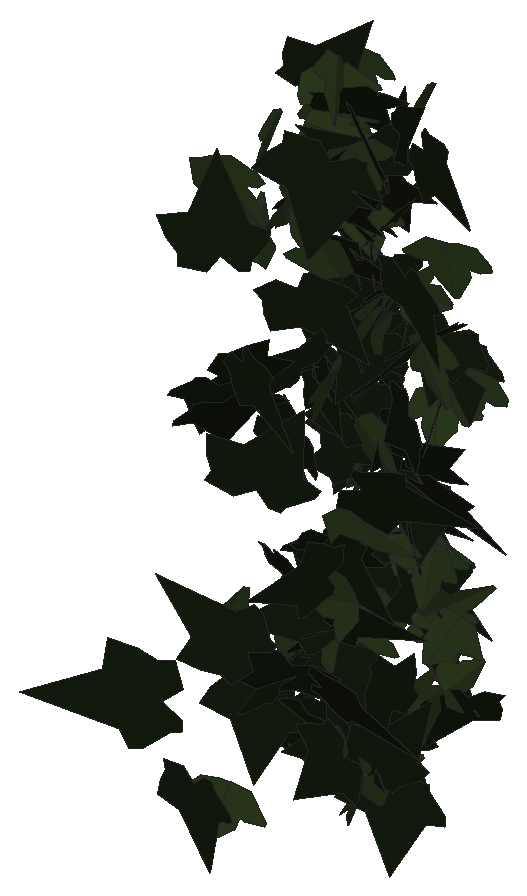
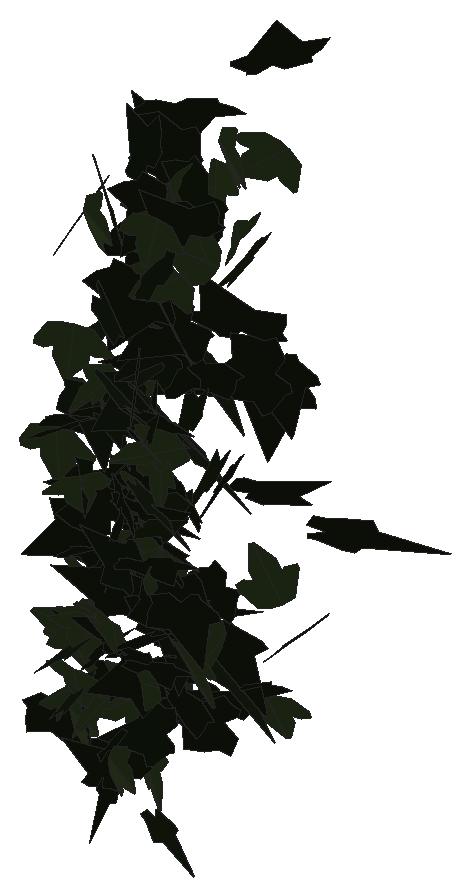
# SketchUp Ruby script. Lengths in inches.
U = 1.inch
M = Sketchup.active_model
def pt(a) = Geom::Point3d.new(a.map { |v| v * U })
def face(e, loops, mat)
  f = e.add_face(loops[0].map { |a| pt(a) })
  loops[1..].each { |l| e.add_face(l.map { |a| pt(a) }).erase! }
  f.material = f.back_material = mat if mat
  f
end
# faces: each face lists its corners as indices into pts; further lists are holes
def faces(e, pts, list, mat = nil) = list.each { |f| face(e, (f[0].is_a?(Array) ? f : [f]).map { |l| l.map { |i| pts[i] } }, mat) }
# xy, xz, yz: faces in a plane at the given z, y or x. An outline is a flat list of corners, or four numbers for a rectangle; further outlines are holes
def ring(l) = l.size == 4 ? [[l[0], l[1]], [l[2], l[1]], [l[2], l[3]], [l[0], l[3]]] : l.each_slice(2).to_a
def flat(e, list, mat, &to3) = list.each { |f| face(e, (f[0].is_a?(Array) ? f : [f]).map { |l| ring(l).map { |u, v| to3.(u, v) } }, mat) }
def xy(e, z, list, mat = nil) = flat(e, list, mat) { |x, y| [x, y, z] }
def xz(e, y, list, mat = nil) = flat(e, list, mat) { |x, z| [x, y, z] }
def yz(e, x, list, mat = nil) = flat(e, list, mat) { |y, z| [x, y, z] }
def lines(e, pts, list) = list.each { |a, b| e.add_line(pt(pts[a]), pt(pts[b])) }
# prism: a flat outline (further loops are holes) pulled along v
def prism(e, loops, v, mat = nil)
  f = face(e, loops, mat); d = Geom::Vector3d.new(v.map { |x| x * U })
  f.pushpull(f.normal.samedirection?(d) ? d.length : -d.length)
end
def box(e, o, s, mat = nil) = prism(e, [[o, [o[0] + s[0], o[1], o[2]], [o[0] + s[0], o[1] + s[1], o[2]], [o[0], o[1] + s[1], o[2]]]], [0, 0, s[2]], mat)
def at(x, y, z, deg = 0) = Geom::Transformation.translation(pt([x, y, z])) * Geom::Transformation.rotation(ORIGIN, Z_AXIS, deg.degrees)
def axes(o, x, y, z) = Geom::Transformation.new([*x, 0, *y, 0, *z, 0, *pt(o).to_a, 1])
def part(name) = M.definitions.add(name)
# library, detail: a bought-in or finely detailed component or shape, given as its bounding box
def library(name, o, s) = part(name).tap { |d| box(d.entities, o, s) }
def detail(e, o, s) = box(e.add_group.entities, o, s)
def put(e, d, t, mat = nil) = e.add_instance(d, t).tap { |i| i.material = mat if mat }
def group(e, t, mat = nil) = e.add_group.tap { |g| g.transformation = t; g.material = mat if mat }.entities
root = M.entities
M.materials.add("1026 AP 7946 SUNNY SIDE UP").color = [254, 231, 186]
M.materials.add("efeu1").color = [18, 25, 13]
M.materials.add("efeu2").color = [43, 57, 29]
c1 = part("ivyleaf_9")
p = [[1.54,2.16,1.25],[1.36,2.04,1.19],[-0.21,0.99,0.68],[-0.71,1.11,0.82],[-0.85,0.86,0.67],[-0.8,0.17,0.21],
  [-0.9,-0.01,0.1],[-0.67,-0.16,-0.02],[-0.08,-0.08,-0.05],[-0.03,-0.6,-0.4],[0.65,-0.88,-0.66],[0.83,-0.6,-0.49],
  [1.29,-0.42,-0.43],[1.8125,-0.07,-0.26],[1.21,0.44,0.15]]
faces(c1.entities,p,[[0,1,2,3,4,5,6,7,8,9,10,11,12,13,14]],"efeu1")
c2 = part("ivyleaf_10")
p = [[0,0.5,-0.03],[-0.0625,2.02,-0.43],[-0.19,2.01,-0.46],[-0.54,1.05,-0.29],[-0.52,0.625,-0.18],[-0.83,0.76,-0.28],
  [-1.16,0.64,-0.33],[-1.15,0.33,-0.24],[-0.77,-0.39,0.02],[-0.3,-0.51,0.16],[0.04,-0.48,0.23],[-0.02,2.01,-0.4375],
  [-0.06,2.01,-0.43],[0.04,-0.49,0.23],[0.67,-0.49,0.14],[1.38,0.36,-0.2],[1.375,0.51,-0.24],[0.81,0.65,-0.19],
  [0.62,0.59,-0.15],[0.6,1.09,-0.28],[0.5,1.23,-0.31]]
faces(c2.entities,p,[[0,1,2,3,4,5,6,7,8,9,10],[11,12,0,13,14,15,16,17,18,19,20]],"efeu2")
put(root,c1,axes([145.76,205.86,279.04],[-0.47575,-0.19404,0.29656],[0.34368,0.19206,0.36975],[-0.42595,0.3717,-0.03289]),"1026 AP 7946 SUNNY SIDE UP")
put(root,c1,axes([144.31,206.23,271.09],[-0.54708,0.00364,0.34311],[-0.51037,-0.11165,-0.34873],[0.11738,-0.46851,0.08287]),"1026 AP 7946 SUNNY SIDE UP")
put(root,c1,axes([144.43,206.95,269.42],[0.03725,-0.39356,0.07755],[0.00838,-0.07733,-0.40663],[0.63067,0.02427,0.00082]),"1026 AP 7946 SUNNY SIDE UP")
put(root,c1,axes([145.21,207.07,271.875],[-0.48703,-0.24842,-0.09158],[-0.13422,-0.03308,0.4079],[-0.39178,0.32015,-0.02589]),"1026 AP 7946 SUNNY SIDE UP")
put(root,c1,axes([145.58,206.94,274.7],[-0.46285,0.03897,0.31305],[0.47694,-0.02004,0.30544],[0.06532,0.42244,-0.01189]),"1026 AP 7946 SUNNY SIDE UP")
put(root,c1,axes([145.11,207.25,276.32],[0.30644,-0.32467,-0.11411],[-0.10935,0.08519,-0.38929],[0.52725,0.20636,-0.01442]),"1026 AP 7946 SUNNY SIDE UP")
put(root,c2,axes([144.17,207.9375,268.78],[0.54849,0.07187,-0.06065],[-0.07976,-0.04619,-0.36545],[-0.12288,0.3508,-0.03352]),"1026 AP 7946 SUNNY SIDE UP")
put(root,c1,axes([146.03,207.875,272.96],[-0.49013,0.29196,0.01363],[-0.04638,-0.01461,-0.43892],[-0.4571,-0.31158,0.02992]),"1026 AP 7946 SUNNY SIDE UP")
put(root,c2,axes([144.07,207.93,278.86],[-0.48766,0.04842,-0.23804],[0.34817,-0.07398,-0.32219],[-0.13,-0.37978,0.03008]),"1026 AP 7946 SUNNY SIDE UP")
put(root,c1,axes([145.76,208.33,279.34],[-0.42337,-0.36772,-0.06327],[0.10281,0.02541,-0.46778],[0.57659,-0.27454,0.03695]),"1026 AP 7946 SUNNY SIDE UP")
put(root,c1,axes([143.9,208.1875,275.16],[0.22014,0.28691,-0.20064],[-0.10461,-0.18569,-0.32942],[-0.53659,0.15391,-0.01809]),"1026 AP 7946 SUNNY SIDE UP")
put(root,c2,axes([143.81,208.3125,271.1],[-0.16669,-0.38173,0.06788],[0.03444,0.06455,0.4085],[-0.60873,0.10818,0.00452]),"1026 AP 7946 SUNNY SIDE UP")
put(root,c1,axes([144,208.15,274.94],[0.22451,0.42748,-0.05577],[-0.0095,-0.05759,-0.46447],[-0.67797,0.14237,-0.01196]),"1026 AP 7946 SUNNY SIDE UP")
put(root,c2,axes([144.9,208.36,278.41],[0.00051,-0.30371,-0.23227],[-0.01416,0.22367,-0.31149],[0.59298,0.0056,-0.00724]),"1026 AP 7946 SUNNY SIDE UP")
put(root,c1,axes([145.49,208.66,278.59],[0.55177,-0.03958,-0.1544],[0.24004,0.02706,0.36155],[-0.04032,-0.38053,0.03951]),"1026 AP 7946 SUNNY SIDE UP")
put(root,c1,axes([145.53,208.88,269.44],[-0.20107,-0.2495,0.28412],[-0.14971,-0.26151,-0.28924],[0.56701,-0.15752,0.02439]),"1026 AP 7946 SUNNY SIDE UP")
put(root,c2,axes([145.59,208.53,277.62],[-0.46288,0.05923,-0.2399],[-0.34125,0.09374,0.3073],[0.16335,0.36367,-0.03781]),"1026 AP 7946 SUNNY SIDE UP")
put(root,c2,axes([144.36,208.45,277.45],[0.03607,0.28011,-0.25507],[-0.00867,0.24987,0.29031],[0.58944,-0.01346,0.01988]),"1026 AP 7946 SUNNY SIDE UP")
put(root,c2,axes([144.3,208.875,279.26],[0.26008,-0.32971,0.16093],[0.09576,-0.14625,-0.38072],[0.56692,0.17596,-0.00952]),"1026 AP 7946 SUNNY SIDE UP")
put(root,c1,axes([145.33,208.82,270.47],[0.4847,-0.14545,0.20611],[0.25549,-0.12369,-0.34983],[0.29464,0.34653,-0.03571]),"1026 AP 7946 SUNNY SIDE UP")
put(root,c1,axes([143.74,208.47,275.19],[0.2872,0.20277,0.34672],[0.42004,0.20638,-0.27718],[-0.45097,0.32136,-0.03737]),"1026 AP 7946 SUNNY SIDE UP")
put(root,c2,axes([145.32,208.93,275.53],[0.13729,-0.39032,0.01038],[-0.00877,-0.01384,-0.41203],[0.61397,0.08708,-0.0082]),"1026 AP 7946 SUNNY SIDE UP")
put(root,c1,axes([143.8125,209.27,269.66],[-0.25448,-0.37842,-0.03572],[0.02966,0.0273,-0.42379],[0.59648,-0.16281,0.00583]),"1026 AP 7946 SUNNY SIDE UP")
put(root,c1,axes([144.39,209.14,270.4],[0.13772,0.24194,-0.33144],[-0.35134,-0.24628,-0.25383],[-0.52857,0.22674,0.08236]),"1026 AP 7946 SUNNY SIDE UP")
put(root,c2,axes([145.12,209.26,269.01],[-0.5227,-0.07691,-0.00354],[-0.01296,0.02236,0.35079],[-0.12033,0.33168,-0.02242]),"1026 AP 7946 SUNNY SIDE UP")
put(root,c1,axes([144.67,209.04,275.37],[-0.2026,0.38144,0.12744],[-0.11869,0.10224,-0.4124],[-0.6182,-0.14464,0.03741]),"1026 AP 7946 SUNNY SIDE UP")
put(root,c1,axes([145.28,209.6,269.28],[-0.20305,-0.12882,0.37096],[-0.35773,-0.28058,-0.18872],[0.48471,-0.26104,0.01612]),"1026 AP 7946 SUNNY SIDE UP")
put(root,c1,axes([144.71,208.93,278.33],[0.19865,0.30027,0.33118],[0.21436,0.28941,-0.33377],[-0.65558,0.18562,-0.00878]),"1026 AP 7946 SUNNY SIDE UP")
put(root,c1,axes([145.39,209.61,279],[0.06704,-0.15701,0.39755],[0.11198,-0.38037,-0.16937],[0.64677,0.08213,-0.01188]),"1026 AP 7946 SUNNY SIDE UP")
put(root,c1,axes([144.125,209.2,270],[-0.26679,0.37063,0.11086],[-0.13798,0.0751,-0.41669],[-0.59002,-0.18515,0.04732]),"1026 AP 7946 SUNNY SIDE UP")
put(root,c1,axes([144.53,209.63,271],[-0.32443,-0.07147,0.26925],[-0.33558,-0.16033,-0.21934],[0.26348,-0.2922,0.05217]),"1026 AP 7946 SUNNY SIDE UP")
put(root,c1,axes([143.95,209.5,269.18],[0.37824,0.07831,-0.31265],[0.38436,0.19345,0.25178],[0.30955,-0.33588,0.0694]),"1026 AP 7946 SUNNY SIDE UP")
put(root,c2,axes([145.13,209.45,271.59],[0.22414,-0.16215,-0.33987],[-0.38624,0.2199,-0.22002],[0.42828,0.28318,-0.02056]),"1026 AP 7946 SUNNY SIDE UP")
put(root,c1,axes([144.56,209.68,269.58],[-0.09341,-0.06056,-0.41655],[0.61625,0.10673,-0.07523],[0.18122,-0.39414,0.04111]),"1026 AP 7946 SUNNY SIDE UP")
put(root,c1,axes([143.92,209.94,273.66],[-0.04302,-0.21817,0.33032],[-0.03709,-0.32115,-0.22819],[0.61031,-0.03489,0.00942]),"1026 AP 7946 SUNNY SIDE UP")
put(root,c1,axes([143.68,209.57,273.91],[0.2436,-0.21098,-0.24254],[-0.23196,0.18213,-0.26845],[0.43807,0.21376,-0.00728]),"1026 AP 7946 SUNNY SIDE UP")
put(root,c1,axes([143.82,209.61,271.72],[0.51088,-0.09389,-0.09989],[-0.15951,-0.00526,-0.34688],[0.13906,0.33887,-0.03093]),"1026 AP 7946 SUNNY SIDE UP")
put(root,c1,axes([145.78,209.46,269.08],[-0.23343,-0.04132,0.38135],[0.48941,0.20559,0.15334],[-0.32239,0.34202,-0.04334]),"1026 AP 7946 SUNNY SIDE UP")
put(root,c2,axes([145.66,209.45,269],[0.0373,-0.03988,-0.41],[0.25163,0.36609,-0.02584],[0.57601,-0.15734,0.03784]),"1026 AP 7946 SUNNY SIDE UP")
put(root,c2,axes([144.02,209.48,270.65],[0.01017,0.03519,0.37263],[-0.22928,0.3314,-0.0286],[-0.52308,-0.14458,0.01978]),"1026 AP 7946 SUNNY SIDE UP")
put(root,c1,axes([145.65,210.02,268.46],[-0.28041,-0.35678,-0.05667],[0.06474,0.03858,-0.41019],[0.56344,-0.18199,0.01893]),"1026 AP 7946 SUNNY SIDE UP")
put(root,c1,axes([144.4,209.81,271.01],[0.3227,-0.027,0.35127],[0.51319,-0.10411,-0.21138],[0.16172,0.38425,-0.03017]),"1026 AP 7946 SUNNY SIDE UP")
put(root,c1,axes([144.65,209.65,270.83],[0.11697,0.38094,0.0121],[0.0188,0.00742,-0.39967],[-0.59889,0.07464,-0.01018]),"1026 AP 7946 SUNNY SIDE UP")
put(root,c1,axes([146,209.8,274.71],[0.17822,-0.0679,-0.40902],[-0.6169,0.07303,-0.12795],[0.14077,0.40601,-0.04287]),"1026 AP 7946 SUNNY SIDE UP")
put(root,c2,axes([144.98,209.875,278.59],[-0.34678,-0.24498,-0.13982],[0.16813,0.0841,-0.33836],[0.40586,-0.24415,0.0207]),"1026 AP 7946 SUNNY SIDE UP")
put(root,c1,axes([143.97,210.28,274.93],[0.00954,-0.18099,0.33189],[0.01933,-0.32296,-0.18845],[0.58212,0.01369,0.00082]),"1026 AP 7946 SUNNY SIDE UP")
put(root,c2,axes([145,210.02,268.3125],[0.11438,-0.36908,-0.04349],[-0.01756,0.03869,-0.3873],[0.5835,0.07351,-0.00313]),"1026 AP 7946 SUNNY SIDE UP")
put(root,c2,axes([144.24,210.02,270.54],[0.47013,-0.22796,-0.13863],[-0.18126,0.06845,-0.38664],[0.37356,0.32011,-0.01314]),"1026 AP 7946 SUNNY SIDE UP")
put(root,c1,axes([145.76,209.72,269.97],[-0.05554,0.2195,0.39031],[-0.20062,0.35715,-0.22407],[-0.65685,-0.12764,0.03543]),"1026 AP 7946 SUNNY SIDE UP")
put(root,c1,axes([144.48,209.95,270.24],[0.02916,-0.23337,-0.28361],[0.0862,0.27296,-0.23412],[0.55929,-0.0299,0.05087]),"1026 AP 7946 SUNNY SIDE UP")
put(root,c1,axes([143.93,209.97,275.94],[-0.09744,-0.15147,-0.35622],[0.2686,0.30025,-0.1657],[0.52794,-0.18072,0.01856]),"1026 AP 7946 SUNNY SIDE UP")
put(root,c2,axes([143.99,209.83,277.73],[0.01936,-0.23384,0.33592],[-0.01861,0.32721,0.24312],[-0.63236,-0.01679,0.00313]),"1026 AP 7946 SUNNY SIDE UP")
put(root,c1,axes([145.15,209.93,273.15],[0.20355,0.08902,-0.38373],[0.36503,0.29514,0.15729],[0.47992,-0.26225,0.04312]),"1026 AP 7946 SUNNY SIDE UP")
put(root,c1,axes([144.23,210.19,271.75],[0.02838,-0.12578,-0.39128],[0.60564,0.10595,-0.0167],[0.16627,-0.36444,0.12762]),"1026 AP 7946 SUNNY SIDE UP")
put(root,c2,axes([144.11,210.52,279.36],[-0.0088,-0.26631,0.26027],[0.29417,-0.22096,-0.23558],[0.49851,0.12569,0.14361]),"1026 AP 7946 SUNNY SIDE UP")
put(root,c1,axes([145.39,210.53,276.39],[0.18805,-0.39477,0.08332],[0.01778,-0.08338,-0.42522],[0.6341,0.11941,-0.01278]),"1026 AP 7946 SUNNY SIDE UP")
put(root,c2,axes([144.67,210.28,272.43],[-0.35841,-0.12128,-0.31798],[0.47763,0.07189,-0.26035],[0.20673,-0.37634,0.05023]),"1026 AP 7946 SUNNY SIDE UP")
put(root,c1,axes([144.01,210.36,271.59],[0.47633,0.22969,-0.08332],[0.0737,0.07378,0.39087],[0.37644,-0.30508,0.0289]),"1026 AP 7946 SUNNY SIDE UP")
put(root,c1,axes([144.91,210.61,277.93],[-0.01925,0.04656,0.39406],[-0.5828,-0.10513,0.00035],[0.16419,-0.36771,0.04743]),"1026 AP 7946 SUNNY SIDE UP")
put(root,c1,axes([143.97,210.46,271.72],[0.09868,0.28641,-0.15481],[-0.05952,-0.14719,-0.30288],[-0.50629,0.07313,0.00543]),"1026 AP 7946 SUNNY SIDE UP")
put(root,c1,axes([145.76,210.5,278.58],[0.31123,-0.27966,-0.22964],[-0.2317,0.16638,-0.35137],[0.51068,0.24592,-0.01946]),"1026 AP 7946 SUNNY SIDE UP")
put(root,c2,axes([144.56,210.73,273.56],[-0.24685,0.12129,-0.32498],[0.3233,-0.24272,-0.20254],[-0.42304,-0.25627,0.03484]),"1026 AP 7946 SUNNY SIDE UP")
put(root,c2,axes([143.88,210.51,278.35],[-0.09647,-0.10232,-0.33067],[0.49996,0.08855,-0.09134],[0.17245,-0.31398,0.07983]),"1026 AP 7946 SUNNY SIDE UP")
put(root,c1,axes([144.3,210.46,279.01],[0.45933,0.225,0.01999],[0.04452,-0.00711,-0.37917],[-0.35213,0.29259,-0.02186]),"1026 AP 7946 SUNNY SIDE UP")
put(root,c1,axes([144.91,210.93,268.77],[-0.06757,0.00095,0.37716],[-0.43366,-0.24251,-0.03412],[0.37859,-0.27761,0.02823]),"1026 AP 7946 SUNNY SIDE UP")
put(root,c1,axes([144.57,210.85,275.05],[-0.52343,-0.10617,-0.11181],[0.17737,-0.00007,-0.35837],[0.15877,-0.34995,0.03175]),"1026 AP 7946 SUNNY SIDE UP")
put(root,c1,axes([145.26,210.87,275.17],[-0.39207,0.13167,-0.25549],[0.22416,-0.22746,-0.27258],[-0.38158,-0.26891,0.10239]),"1026 AP 7946 SUNNY SIDE UP")
put(root,c2,axes([144.07,210.67,278.67],[-0.49889,-0.13328,-0.12052],[0.18611,0.01734,-0.35323],[0.20661,-0.33746,0.02716]),"1026 AP 7946 SUNNY SIDE UP")
put(root,c1,axes([145,210.84,278.43],[-0.01106,0.18696,0.33902],[0.03223,-0.32741,0.19078],[0.59281,0.02129,-0.00405]),"1026 AP 7946 SUNNY SIDE UP")
put(root,c1,axes([143.76,210.68,276.27],[0.44772,-0.04096,0.22212],[0.32677,-0.06441,-0.29539],[0.11207,0.35145,-0.0261]),"1026 AP 7946 SUNNY SIDE UP")
put(root,c1,axes([143.54,210.9,274.05],[-0.0954,-0.09302,-0.31281],[0.49707,-0.04159,-0.05228],[-0.03853,-0.30632,0.1001]),"1026 AP 7946 SUNNY SIDE UP")
put(root,c2,axes([145.56,210.84,271.85],[0.51756,-0.12644,0.0806],[0.09817,-0.05685,-0.36227],[0.21285,0.33368,-0.02889]),"1026 AP 7946 SUNNY SIDE UP")
put(root,c2,axes([145.48,210.88,275.15],[-0.40593,0.12352,-0.24827],[0.22417,-0.22214,-0.27513],[-0.36319,-0.27517,0.10767]),"1026 AP 7946 SUNNY SIDE UP")
put(root,c2,axes([143.85,210.74,279.01],[0.37747,0.26321,0.07887],[0.09615,0.04575,-0.36644],[-0.41949,0.24733,-0.01302]),"1026 AP 7946 SUNNY SIDE UP")
put(root,c2,axes([144.58,210.94,275.51],[0.07344,-0.31547,0.15962],[0.01189,-0.15717,-0.32914],[0.55376,0.04521,-0.0141]),"1026 AP 7946 SUNNY SIDE UP")
put(root,c2,axes([145.59,211.08,269.43],[0.16058,-0.25121,0.26359],[0.13976,-0.24153,-0.2807],[0.54787,0.13524,-0.00565]),"1026 AP 7946 SUNNY SIDE UP")
put(root,c1,axes([143.78,211,277.22],[-0.33778,0.04735,-0.27606],[0.38916,-0.10875,-0.2246],[-0.17888,-0.326,0.03266]),"1026 AP 7946 SUNNY SIDE UP")
put(root,c1,axes([144.66,211.17,273.45],[0.06282,-0.12382,-0.3245],[0.34722,-0.22992,0.12089],[-0.40194,-0.21797,0.05371]),"1026 AP 7946 SUNNY SIDE UP")
put(root,c2,axes([145.85,210.97,270.77],[0.51676,-0.04807,-0.07862],[-0.12212,-0.00622,-0.34176],[0.0714,0.33727,-0.0155]),"1026 AP 7946 SUNNY SIDE UP")
put(root,c1,axes([144.22,210.78,272.96],[-0.44956,0.02529,-0.15322],[-0.22604,0.05203,0.29382],[0.0727,0.31812,-0.03395]),"1026 AP 7946 SUNNY SIDE UP")
put(root,c2,axes([144.3,210.88,270.2],[0.31444,-0.02229,-0.24567],[0.37596,0.03386,0.2036],[0.0185,-0.30928,0.03815]),"1026 AP 7946 SUNNY SIDE UP")
put(root,c1,axes([145.0625,210.99,273.2],[0.53017,0.05322,-0.08796],[0.12345,0.0492,0.35006],[0.09956,-0.34439,0.03431]),"1026 AP 7946 SUNNY SIDE UP")
put(root,c2,axes([144.8,210.67,275.32],[0.07109,0.04488,0.37767],[-0.26565,0.33067,-0.01832],[-0.51599,-0.16406,0.06146]),"1026 AP 7946 SUNNY SIDE UP")
put(root,c1,axes([144.4,210.96,275.69],[-0.48469,0.22881,0.00825],[-0.03626,-0.01985,-0.39441],[-0.35811,-0.30768,0.02878]),"1026 AP 7946 SUNNY SIDE UP")
put(root,c1,axes([143.55,210.82,278.875],[-0.21764,-0.04594,0.35003],[0.50478,0.11213,0.15088],[-0.19051,0.34959,-0.0001]),"1026 AP 7946 SUNNY SIDE UP")
put(root,c1,axes([145.21,211.15,272.64],[-0.24366,-0.3105,-0.04862],[0.08242,0.02434,-0.35545],[0.48649,-0.15964,0.03587]),"1026 AP 7946 SUNNY SIDE UP")
put(root,c2,axes([144.11,210.95,276.89],[0.47827,0.13695,0.11353],[0.14085,0.06694,-0.34244],[-0.23693,0.31624,0.0256]),"1026 AP 7946 SUNNY SIDE UP")
put(root,c1,axes([143.9,211.03,269.63],[0.45616,-0.18389,0.12766],[0.14601,-0.08644,-0.35363],[0.31764,0.30382,-0.02078]),"1026 AP 7946 SUNNY SIDE UP")
put(root,c1,axes([143.5625,210.85,277.22],[0.59431,0.05802,0.05016],[0.07988,-0.01268,-0.39347],[-0.08789,0.38083,-0.01846]),"1026 AP 7946 SUNNY SIDE UP")
put(root,c1,axes([145.19,210.88,272.19],[0.29603,-0.15259,-0.28384],[-0.38165,0.13269,-0.24657],[0.31373,0.30541,-0.03212]),"1026 AP 7946 SUNNY SIDE UP")
put(root,c2,axes([143.79,210.99,277.98],[-0.40722,-0.02577,-0.22735],[0.34887,-0.04321,-0.26346],[-0.01357,-0.3374,0.04909]),"1026 AP 7946 SUNNY SIDE UP")
put(root,c2,axes([145.4375,210.74,269.53],[-0.02531,0.14279,0.33144],[-0.10717,0.31387,-0.14556],[-0.54181,-0.06875,0.01331]),"1026 AP 7946 SUNNY SIDE UP")
put(root,c2,axes([143.97,211.26,272.63],[-0.08248,0.02447,0.36119],[0.26329,-0.30977,0.04629],[0.48564,0.1721,0.03625]),"1026 AP 7946 SUNNY SIDE UP")
put(root,c1,axes([145.11,210.84,268.34],[0.11734,-0.1142,-0.35423],[-0.37647,0.24706,-0.13688],[0.4263,0.24962,-0.02338]),"1026 AP 7946 SUNNY SIDE UP")
put(root,c1,axes([144.45,210.89,277.56],[0.53975,0.15269,-0.09416],[-0.11336,-0.06429,-0.38629],[-0.25659,0.34959,-0.02741]),"1026 AP 7946 SUNNY SIDE UP")
put(root,c1,axes([145.43,210.99,272.83],[0.56214,-0.06916,0.06268],[0.08298,-0.04798,-0.37351],[0.11922,0.35952,-0.03557]),"1026 AP 7946 SUNNY SIDE UP")
put(root,c1,axes([145.09,211.32,270.77],[-0.14162,-0.1383,0.29329],[-0.18917,-0.2597,-0.17023],[0.46153,-0.14888,0.02023]),"1026 AP 7946 SUNNY SIDE UP")
put(root,c1,axes([143.8,211.05,276.65],[0.51721,-0.14524,0.00929],[-0.00501,-0.0315,-0.36931],[0.22884,0.32757,-0.02908]),"1026 AP 7946 SUNNY SIDE UP")
put(root,c1,axes([143.96,211.08,276.47],[0.36066,-0.2587,-0.04126],[0.02062,0.06262,-0.35191],[0.41076,0.22401,0.05389]),"1026 AP 7946 SUNNY SIDE UP")
put(root,c1,axes([144.5,211.33,271.125],[-0.25782,-0.11169,0.25284],[-0.21658,-0.21308,-0.19543],[0.36556,-0.20501,0.06253]),"1026 AP 7946 SUNNY SIDE UP")
put(root,c1,axes([144.26,211.12,274.83],[0.24621,-0.2966,-0.13416],[-0.11759,0.10572,-0.34452],[0.4945,0.17282,-0.01513]),"1026 AP 7946 SUNNY SIDE UP")
put(root,c1,axes([143.51,211.1,273.85],[0.41816,-0.23457,-0.05105],[-0.02243,0.05642,-0.36344],[0.37588,0.26432,0.03511]),"1026 AP 7946 SUNNY SIDE UP")
put(root,c1,axes([145.62,210.89,274.04],[-0.06993,0.00517,-0.3637],[-0.44776,0.2099,0.04135],[0.32831,0.28737,-0.02108]),"1026 AP 7946 SUNNY SIDE UP")
put(root,c1,axes([145.98,211.15,269.54],[0.06279,0.23681,-0.25137],[-0.03622,-0.24459,-0.2485],[-0.53496,0.04436,-0.01268]),"1026 AP 7946 SUNNY SIDE UP")
put(root,c1,axes([144.95,211.23,277.29],[-0.36515,0.20233,-0.22242],[0.19279,-0.18556,-0.31443],[-0.42489,-0.25808,0.04848]),"1026 AP 7946 SUNNY SIDE UP")
put(root,c1,axes([145.38,210.95,275.23],[0.03991,0.37515,0.00943],[-0.02357,0.00805,-0.38698],[-0.58952,0.02508,0.01611]),"1026 AP 7946 SUNNY SIDE UP")
put(root,c1,axes([143.74,211.41,278.15],[0.04657,-0.2232,0.30832],[0.08293,-0.296,-0.23354],[0.58279,0.05995,0.0086]),"1026 AP 7946 SUNNY SIDE UP")
put(root,c2,axes([145.63,210.99,270.89],[-0.08143,-0.2182,0.28163],[0.17518,0.25298,0.2302],[-0.52296,0.11872,0.03326]),"1026 AP 7946 SUNNY SIDE UP")
put(root,c1,axes([144.35,211.05,273.55],[-0.60133,-0.06046,-0.09824],[-0.15489,0.01654,0.3977],[-0.08583,0.39371,-0.02943]),"1026 AP 7946 SUNNY SIDE UP")
put(root,c1,axes([144.48,211.28,275.21],[-0.52069,0.06697,-0.16437],[0.23381,-0.06766,-0.34675],[-0.14023,-0.36147,0.03219]),"1026 AP 7946 SUNNY SIDE UP")
put(root,c1,axes([144.74,211.04,268.6],[-0.09697,-0.00409,0.33083],[0.49512,0.06369,0.0635],[-0.09954,0.32076,-0.00643]),"1026 AP 7946 SUNNY SIDE UP")
put(root,c1,axes([143.93,211.13,268.09],[-0.23428,0.24696,-0.03897],[0.01047,-0.04173,-0.29694],[-0.39305,-0.14831,0.01532]),"1026 AP 7946 SUNNY SIDE UP")
put(root,c2,axes([143.93,211.125,274.625],[-0.45804,0.20567,0.09063],[-0.15703,0.00758,-0.36369],[-0.31393,-0.30386,0.04968]),"1026 AP 7946 SUNNY SIDE UP")
put(root,c2,axes([145.05,211.4,278.89],[0.21074,-0.27794,0.20628],[0.10488,-0.19145,-0.31838],[0.52981,0.14845,-0.01903]),"1026 AP 7946 SUNNY SIDE UP")
put(root,c1,axes([144.04,211.375,275.6],[-0.48842,-0.11911,-0.08059],[0.13587,-0.01027,-0.34036],[0.17744,-0.31999,0.03879]),"1026 AP 7946 SUNNY SIDE UP")
put(root,c1,axes([145.45,211.44,275.125],[-0.27536,-0.31641,0.01358],[0.01395,-0.02201,-0.3722],[0.49788,-0.17438,0.01794]),"1026 AP 7946 SUNNY SIDE UP")
put(root,c1,axes([144.4,210.94,275.52],[0.24269,0.20727,0.26953],[0.18839,0.23326,-0.26301],[-0.48832,0.193,0.03249]),"1026 AP 7946 SUNNY SIDE UP")
put(root,c1,axes([144.84,211.23,275.9],[-0.4093,0.25739,-0.03864],[0.01538,-0.0454,-0.37649],[-0.40905,-0.25926,0.02451]),"1026 AP 7946 SUNNY SIDE UP")
put(root,c2,axes([143.97,211.33,270.65],[-0.14723,0.04087,-0.29056],[0.36801,-0.1588,-0.10459],[-0.25634,-0.25146,0.01673]),"1026 AP 7946 SUNNY SIDE UP")
put(root,c1,axes([143.88,211.42,271.07],[-0.35257,-0.19719,-0.04359],[0.07975,0.00439,-0.30604],[0.30655,-0.22793,0.02949]),"1026 AP 7946 SUNNY SIDE UP")
put(root,c2,axes([145.79,211.02,269.76],[0.11096,0.02399,-0.3497],[0.1447,0.33255,0.04585],[0.51537,-0.09854,0.06242]),"1026 AP 7946 SUNNY SIDE UP")
put(root,c2,axes([145.39,211.37,270.35],[0.527,-0.04196,0.04436],[0.06002,-0.04163,-0.3462],[0.07338,0.33537,-0.0354]),"1026 AP 7946 SUNNY SIDE UP")
put(root,c1,axes([144.43,211.18,272.54],[0.16228,0.29701,-0.00889],[-0.03389,0.01837,0.32289],[0.46607,-0.10208,0.02658]),"1026 AP 7946 SUNNY SIDE UP")
put(root,c2,axes([144.51,211.46,269.05],[0.11913,-0.2724,0.16677],[0.05626,-0.15962,-0.29212],[0.49632,0.08348,-0.00692]),"1026 AP 7946 SUNNY SIDE UP")
put(root,c1,axes([144.3,211.15,276.41],[0.15111,-0.09345,-0.3361],[-0.43315,0.17561,-0.13461],[0.31028,0.29067,-0.02423]),"1026 AP 7946 SUNNY SIDE UP")
put(root,c1,axes([143.84,211.49,275.36],[-0.11267,0.04849,0.31451],[-0.05246,-0.31251,0.04128],[0.4828,-0.02264,0.07788]),"1026 AP 7946 SUNNY SIDE UP")
put(root,c1,axes([144.48,211.37,272.14],[0.27988,-0.10804,0.27559],[0.35001,-0.14966,-0.21524],[0.29,0.28491,-0.00619]),"1026 AP 7946 SUNNY SIDE UP")
put(root,c1,axes([143.875,211.52,273.02],[-0.38714,-0.24162,-0.0134],[0.05014,-0.01597,-0.35377],[0.37704,-0.24597,0.03329]),"1026 AP 7946 SUNNY SIDE UP")
put(root,c1,axes([145.3125,211.36,270.12],[0.27295,-0.27499,-0.09212],[-0.09738,0.06465,-0.33417],[0.44336,0.18349,-0.01669]),"1026 AP 7946 SUNNY SIDE UP")
put(root,c1,axes([145.62,211.54,274.88],[-0.11348,-0.34035,0.01293],[0.06936,-0.02402,-0.35512],[0.53114,-0.06958,0.04914]),"1026 AP 7946 SUNNY SIDE UP")
put(root,c2,axes([145.52,211.35,276.53],[-0.53326,-0.1173,-0.01278],[0.0375,-0.03325,-0.36766],[0.18153,-0.33771,0.03841]),"1026 AP 7946 SUNNY SIDE UP")
put(root,c2,axes([145.83,211.39,274.57],[-0.55662,-0.05607,0.03006],[-0.02365,-0.08827,-0.35932],[0.09677,-0.34408,0.08508]),"1026 AP 7946 SUNNY SIDE UP")
put(root,c2,axes([145.06,211.09,275.76],[-0.01123,0.16463,0.33601],[-0.03055,0.32465,-0.16784],[-0.57235,-0.02056,0.00236]),"1026 AP 7946 SUNNY SIDE UP")
put(root,c1,axes([144.12,211.35,274.18],[-0.36174,0.2386,-0.01908],[-0.004,-0.03,-0.34083],[-0.37645,-0.22895,0.02196]),"1026 AP 7946 SUNNY SIDE UP")
put(root,c2,axes([143.62,211.23,275.05],[0.15123,0.12706,0.34854],[0.34518,0.25663,-0.16242],[-0.45008,0.23951,-0.00746]),"1026 AP 7946 SUNNY SIDE UP")
put(root,c2,axes([143.8125,211.4,279.11],[-0.51877,0.02889,-0.01184],[0.01369,-0.03355,-0.33971],[-0.04703,-0.32841,0.03171]),"1026 AP 7946 SUNNY SIDE UP")
put(root,c2,axes([145.24,211.46,273.99],[0.32288,0.28144,-0.06479],[-0.03773,-0.06223,-0.35884],[-0.45244,0.20604,-0.01632]),"1026 AP 7946 SUNNY SIDE UP")
put(root,c1,axes([144.17,211.12,270.69],[-0.01905,0.19626,-0.31848],[-0.13406,0.30044,0.20097],[0.56149,0.07839,0.03718]),"1026 AP 7946 SUNNY SIDE UP")
put(root,c1,axes([144.26,211.58,274.03],[-0.11585,-0.03366,-0.31263],[0.46579,-0.08274,-0.06516],[-0.1151,-0.30093,0.05097]),"1026 AP 7946 SUNNY SIDE UP")
put(root,c2,axes([144.77,211.54,271.63],[-0.37299,0.07629,-0.2002],[0.20023,-0.18096,-0.23385],[-0.26093,-0.2479,0.10673]),"1026 AP 7946 SUNNY SIDE UP")
put(root,c2,axes([145.02,211.43,271.43],[0.43969,0.17863,0.09149],[0.11606,0.04754,-0.34156],[-0.29065,0.28921,0.00202]),"1026 AP 7946 SUNNY SIDE UP")
put(root,c2,axes([144.98,211.44,271.5],[0.51524,0.0538,0.09184],[0.12334,0.06456,-0.33793],[-0.10705,0.33331,0.0527]),"1026 AP 7946 SUNNY SIDE UP")
put(root,c1,axes([145.28,211.32,271.12],[-0.5047,0.10628,0.01242],[0.02133,0.00455,0.34824],[0.16673,0.32115,-0.00695]),"1026 AP 7946 SUNNY SIDE UP")
put(root,c1,axes([145.19,211.41,271.11],[0.32608,-0.21978,-0.15375],[-0.07939,0.15172,-0.3041],[0.409,0.20467,0.06355]),"1026 AP 7946 SUNNY SIDE UP")
